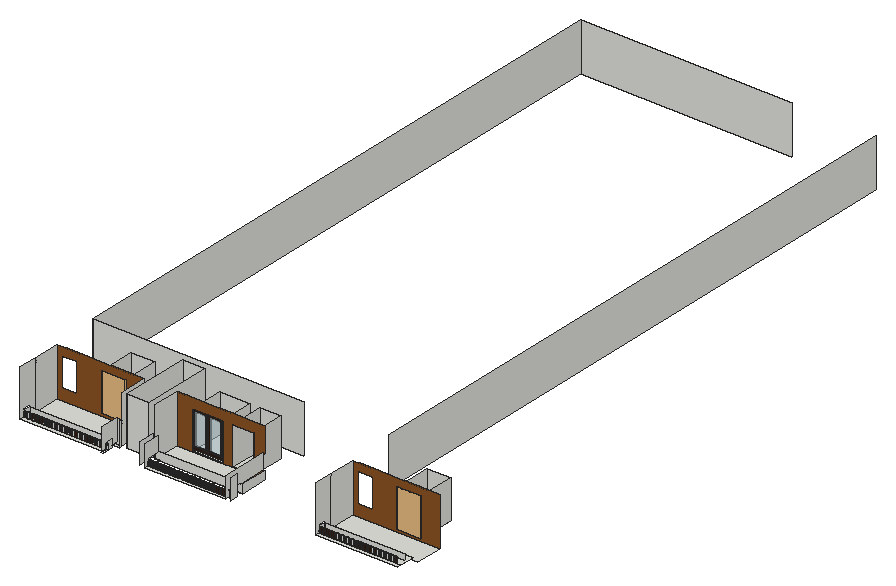
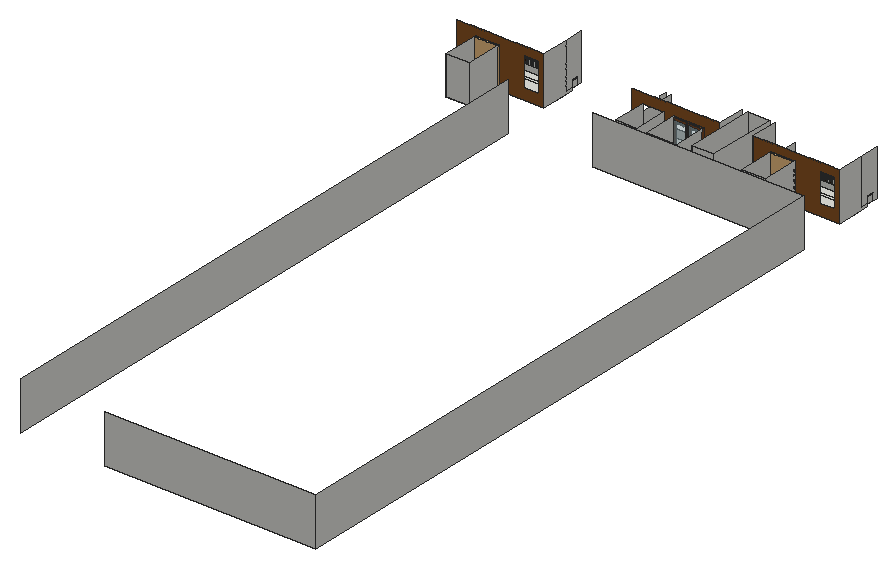
# SketchUp Ruby script. Lengths in inches.
U = 1.inch
M = Sketchup.active_model
def pt(a) = Geom::Point3d.new(a.map { |v| v * U })
def face(e, loops, mat)
  f = e.add_face(loops[0].map { |a| pt(a) })
  loops[1..].each { |l| e.add_face(l.map { |a| pt(a) }).erase! }
  f.material = f.back_material = mat if mat
  f
end
# faces: each face lists its corners as indices into pts; further lists are holes
def faces(e, pts, list, mat = nil) = list.each { |f| face(e, (f[0].is_a?(Array) ? f : [f]).map { |l| l.map { |i| pts[i] } }, mat) }
# xy, xz, yz: faces in a plane at the given z, y or x. An outline is a flat list of corners, or four numbers for a rectangle; further outlines are holes
def ring(l) = l.size == 4 ? [[l[0], l[1]], [l[2], l[1]], [l[2], l[3]], [l[0], l[3]]] : l.each_slice(2).to_a
def flat(e, list, mat, &to3) = list.each { |f| face(e, (f[0].is_a?(Array) ? f : [f]).map { |l| ring(l).map { |u, v| to3.(u, v) } }, mat) }
def xy(e, z, list, mat = nil) = flat(e, list, mat) { |x, y| [x, y, z] }
def xz(e, y, list, mat = nil) = flat(e, list, mat) { |x, z| [x, y, z] }
def yz(e, x, list, mat = nil) = flat(e, list, mat) { |y, z| [x, y, z] }
def lines(e, pts, list) = list.each { |a, b| e.add_line(pt(pts[a]), pt(pts[b])) }
# prism: a flat outline (further loops are holes) pulled along v
def prism(e, loops, v, mat = nil)
  f = face(e, loops, mat); d = Geom::Vector3d.new(v.map { |x| x * U })
  f.pushpull(f.normal.samedirection?(d) ? d.length : -d.length)
end
def box(e, o, s, mat = nil) = prism(e, [[o, [o[0] + s[0], o[1], o[2]], [o[0] + s[0], o[1] + s[1], o[2]], [o[0], o[1] + s[1], o[2]]]], [0, 0, s[2]], mat)
def at(x, y, z, deg = 0) = Geom::Transformation.translation(pt([x, y, z])) * Geom::Transformation.rotation(ORIGIN, Z_AXIS, deg.degrees)
def axes(o, x, y, z) = Geom::Transformation.new([*x, 0, *y, 0, *z, 0, *pt(o).to_a, 1])
def part(name) = M.definitions.add(name)
# library, detail: a bought-in or finely detailed component or shape, given as its bounding box
def library(name, o, s) = part(name).tap { |d| box(d.entities, o, s) }
def detail(e, o, s) = box(e.add_group.entities, o, s)
def put(e, d, t, mat = nil) = e.add_instance(d, t).tap { |i| i.material = mat if mat }
def group(e, t, mat = nil) = e.add_group.tap { |g| g.transformation = t; g.material = mat if mat }.entities
root = M.entities
M.materials.add("[Translucent Glass Safety]").color = [204, 235, 244]
M.materials["[Translucent Glass Safety]"].alpha = 0.5
M.materials.add("[Wood Floor Parquet]").color = [140, 85, 37]
M.materials.add("[Wood Veneer 01]").color = [51, 28, 15]
M.materials.add("[Wood Veneer 01]1").color = [120, 70, 37]
c1 = library("元件\#5",[-4.39,0,0],[5.37,35.83,90.55])
c2 = part("Component\#1")
xy(c2.entities,0,[[0,0,6,48]],"[Wood Veneer 01]1")
xy(c2.entities,4,[[0,4,1.8125,44],[1.8125,4,6,44]])
xy(c2.entities,80,[[0,4,1.8125,44],[1.8125,4,6,44]])
xy(c2.entities,84,[[0,0,6,48]],"[Wood Veneer 01]1")
xz(c2.entities,0,[[0,0,6,84]],"[Wood Veneer 01]1")
xz(c2.entities,4,[[0,4,1.8125,80],[1.8125,4,6,80]])
xz(c2.entities,44,[[0,4,1.8125,80],[1.8125,4,6,80]])
xz(c2.entities,48,[[0,0,6,84]],"[Wood Veneer 01]1")
yz(c2.entities,0,[[[0,0,48,84],[4,4,44,80]]],"[Wood Veneer 01]1")
yz(c2.entities,1.8125,[[4,4,44,80]],"[Translucent Glass Safety]")
yz(c2.entities,6,[[[0,0,48,84],[4,4,44,80]]],"[Wood Veneer 01]")
c3 = part("Group\#3")
put(c3.entities,c2,at(0,0,0),"[Wood Veneer 01]")
g1 = group(c3.entities,at(0,48,0),"[Wood Veneer 01]")
xy(g1,0,[[0,0,6,48]],"[Wood Veneer 01]1")
xy(g1,4,[[0,4,1.8125,44],[1.8125,4,6,44]])
xy(g1,80,[[0,4,1.8125,44],[1.8125,4,6,44]])
xy(g1,84,[[0,0,6,48]],"[Wood Veneer 01]1")
xz(g1,0,[[0,0,6,84]],"[Wood Veneer 01]1")
xz(g1,4,[[0,4,1.8125,80],[1.8125,4,6,80]])
xz(g1,44,[[0,4,1.8125,80],[1.8125,4,6,80]])
xz(g1,48,[[0,0,6,84]],"[Wood Veneer 01]1")
yz(g1,0,[[[0,0,48,84],[4,4,44,80]]],"[Wood Veneer 01]1")
yz(g1,1.8125,[[4,4,44,80]],"[Translucent Glass Safety]")
yz(g1,6,[[[0,0,48,84],[4,4,44,80]]],"[Wood Veneer 01]")
xy(root,134.6875,[[100.18,275.15,298.48,293.45],[833.74,275.15,1032.04,293.45],[298.48,286.21,315.43,293.45],[100.18,293.45,315.43,361.27],[328.03,293.45,382.74,465.02],
  [396.57,293.45,614.76,361.27],[833.74,293.45,1049,361.27]])
xy(root,135.5625,[[435.49,361.27,509.74,445.08],[534.92,361.27,587.67,445.08]])
xy(root,140.625,[[100.18,246.64,303.35,256.84],[409.32,246.64,609.07,246.64,609.07,256.84,412.47,256.84,412.47,255.72,409.32,255.72],[833.74,246.64,1036.91,256.84],[100.18,256.84,303.35,256.84,303.35,293.45,298.48,293.45,298.48,293.46,100.18,293.46],[833.74,256.84,1036.91,256.84,1036.91,293.45,1032.04,293.45,1032.04,293.46,833.74,293.46]])
xy(root,140.625,[[409.32,255.72,412.47,256.78]],"[Wood Veneer 01]")
xy(root,141,[[210.43,361.27,269.1,452.7],[943.99,361.27,1002.66,452.7]])
xz(root,255.72,[[409.32,140.625,412.47,154.75],[413.32,140.625,416.47,154.75],[417.32,140.625,420.47,154.75],[421.32,140.625,424.47,154.75],[425.32,140.625,428.47,154.75],
  [429.32,140.625,432.47,154.75],[433.32,140.625,436.47,154.75],[437.32,140.625,440.47,154.75],[441.32,140.625,444.47,154.75],[445.32,140.625,448.47,154.75],
  [449.32,140.625,452.47,154.75],[453.32,140.625,456.47,154.75],[457.32,140.625,460.47,154.75],[461.32,140.625,464.47,154.75],[465.32,140.625,468.47,154.75],
  [469.32,140.625,472.47,154.75],[473.32,140.625,476.47,154.75],[477.32,140.625,480.47,154.75],[481.32,140.625,484.47,154.75],[485.32,140.625,488.47,154.75],
  [489.32,140.625,492.47,154.75],[493.32,140.625,496.47,154.75],[497.32,140.625,500.47,154.75],[501.32,140.625,504.47,154.75],[505.32,140.625,508.47,154.75],
  [509.32,140.625,512.47,154.75],[513.32,140.625,516.47,154.75],[517.32,140.625,520.47,154.75],[521.32,140.625,524.47,154.75],[525.32,140.625,528.47,154.75],
  [529.32,140.625,532.47,154.75],[533.32,140.625,536.47,154.75],[537.32,140.625,540.47,154.75],[541.32,140.625,544.47,154.75],[545.32,140.625,548.47,154.75],
  [549.32,140.625,552.47,154.75],[553.32,140.625,556.47,154.75],[557.32,140.625,560.47,154.75],[561.32,140.625,564.47,154.75],[565.32,140.625,568.47,154.75],
  [569.32,140.625,572.47,154.75],[573.32,140.625,576.47,154.75],[577.32,140.625,580.47,154.75],[581.32,140.625,584.47,154.75],[585.32,140.625,588.47,154.75],
  [589.32,140.625,592.47,154.75],[593.32,140.625,596.47,154.75],[597.32,140.625,600.47,154.75],[601.32,140.625,604.47,154.75],[605.32,140.625,608.47,154.75],
  [609.32,140.625,612.47,154.75]],"[Wood Veneer 01]")
xz(root,256.78,[[409.32,140.625,412.47,154.75]],"[Wood Veneer 01]")
xz(root,256.84,[[103.45,140.625,104.3,154.75],[107.58,140.625,108.43,154.75],[111.7,140.625,112.55,154.75],[115.83,140.625,116.68,154.75],[119.95,140.625,120.8,154.75],
  [124.08,140.625,124.93,154.75],[128.2,140.625,129.05,154.75],[132.33,140.625,133.18,154.75],[136.45,140.625,137.3,154.75],[140.58,140.625,141.43,154.75],
  [144.7,140.625,145.55,154.75],[148.83,140.625,149.68,154.75],[152.95,140.625,153.8,154.75],[157.08,140.625,157.93,154.75],[161.2,140.625,162.05,154.75],
  [165.33,140.625,166.18,154.75],[169.45,140.625,170.3,154.75],[173.58,140.625,174.43,154.75],[177.7,140.625,178.55,154.75],[181.83,140.625,182.68,154.75],
  [185.95,140.625,186.8,154.75],[190.08,140.625,190.93,154.75],[194.2,140.625,195.05,154.75],[198.33,140.625,199.18,154.75],[202.45,140.625,203.3,154.75],
  [206.58,140.625,207.43,154.75],[210.7,140.625,211.55,154.75],[214.83,140.625,215.68,154.75],[218.95,140.625,219.8,154.75],[223.08,140.625,223.93,154.75],
  [227.2,140.625,228.05,154.75],[231.33,140.625,232.18,154.75],[235.45,140.625,236.3,154.75],[239.58,140.625,240.43,154.75],[243.7,140.625,244.55,154.75],
  [247.83,140.625,248.68,154.75],[251.95,140.625,252.8,154.75],[256.08,140.625,256.93,154.75],[260.2,140.625,261.05,154.75],[264.33,140.625,265.18,154.75],
  [268.45,140.625,269.3,154.75],[272.58,140.625,273.43,154.75],[276.7,140.625,277.55,154.75],[280.83,140.625,281.68,154.75],[284.95,140.625,285.8,154.75],
  [289.08,140.625,289.93,154.75],[293.2,140.625,294.05,154.75],[297.33,140.625,298.18,154.75],[301.45,140.625,302.3,154.75],[303.41,140.625,305.58,154.75],
  [306.43,140.625,309.7,154.75],[412.47,140.625,609.07,154.75],[609.07,140.625,614.76,154.75],[837.02,140.625,837.86,154.75],[841.14,140.625,841.99,154.75],
  [845.27,140.625,846.11,154.75],[849.39,140.625,850.24,154.75],[853.52,140.625,854.36,154.75],[857.64,140.625,858.49,154.75],[861.77,140.625,862.61,154.75],
  [865.89,140.625,866.74,154.75],[870.02,140.625,870.86,154.75],[874.14,140.625,874.99,154.75],[878.27,140.625,879.11,154.75],[882.39,140.625,883.24,154.75],
  [886.52,140.625,887.36,154.75],[890.64,140.625,891.49,154.75],[894.77,140.625,895.61,154.75],[898.89,140.625,899.74,154.75],[903.02,140.625,903.86,154.75],
  [907.14,140.625,907.99,154.75],[911.27,140.625,912.11,154.75],[915.39,140.625,916.24,154.75],[919.52,140.625,920.36,154.75],[923.64,140.625,924.49,154.75],
  [927.77,140.625,928.61,154.75],[931.89,140.625,932.74,154.75],[936.02,140.625,936.86,154.75],[940.14,140.625,940.99,154.75],[944.27,140.625,945.11,154.75],
  [948.39,140.625,949.24,154.75],[952.52,140.625,953.36,154.75],[956.64,140.625,957.49,154.75],[960.77,140.625,961.61,154.75],[964.89,140.625,965.74,154.75],
  [969.02,140.625,969.86,154.75],[973.14,140.625,973.99,154.75],[977.27,140.625,978.11,154.75],[981.39,140.625,982.24,154.75],[985.52,140.625,986.36,154.75],
  [989.64,140.625,990.49,154.75],[993.77,140.625,994.61,154.75],[997.89,140.625,998.74,154.75],[1002.02,140.625,1002.86,154.75],[1006.14,140.625,1006.99,154.75],
  [1010.27,140.625,1011.11,154.75],[1014.39,140.625,1015.24,154.75],[1018.52,140.625,1019.36,154.75],[1022.64,140.625,1023.49,154.75]])
xz(root,256.84,[[100.18,140.625,103.45,154.75],[104.3,140.625,107.58,154.75],[108.43,140.625,111.7,154.75],[112.55,140.625,115.83,154.75],[116.68,140.625,119.95,154.75],
  [120.8,140.625,124.08,154.75],[124.93,140.625,128.2,154.75],[129.05,140.625,132.33,154.75],[133.18,140.625,136.45,154.75],[137.3,140.625,140.58,154.75],
  [141.43,140.625,144.7,154.75],[145.55,140.625,148.83,154.75],[149.68,140.625,152.95,154.75],[153.8,140.625,157.08,154.75],[157.93,140.625,161.2,154.75],
  [162.05,140.625,165.33,154.75],[166.18,140.625,169.45,154.75],[170.3,140.625,173.58,154.75],[174.43,140.625,177.7,154.75],[178.55,140.625,181.83,154.75],
  [182.68,140.625,185.95,154.75],[186.8,140.625,190.08,154.75],[190.93,140.625,194.2,154.75],[195.05,140.625,198.33,154.75],[199.18,140.625,202.45,154.75],
  [203.3,140.625,206.58,154.75],[207.43,140.625,210.7,154.75],[211.55,140.625,214.83,154.75],[215.68,140.625,218.95,154.75],[219.8,140.625,223.08,154.75],
  [223.93,140.625,227.2,154.75],[228.05,140.625,231.33,154.75],[232.18,140.625,235.45,154.75],[236.3,140.625,239.58,154.75],[240.43,140.625,243.7,154.75],
  [244.55,140.625,247.83,154.75],[248.68,140.625,251.95,154.75],[252.8,140.625,256.08,154.75],[256.93,140.625,260.2,154.75],[261.05,140.625,264.33,154.75],
  [265.18,140.625,268.45,154.75],[269.3,140.625,272.58,154.75],[273.43,140.625,276.7,154.75],[277.55,140.625,280.83,154.75],[281.68,140.625,284.95,154.75],
  [285.8,140.625,289.08,154.75],[289.93,140.625,293.2,154.75],[294.05,140.625,297.33,154.75],[298.18,140.625,301.45,154.75],[302.3,140.625,303.41,154.75],
  [833.74,140.625,837.02,154.75],[837.86,140.625,841.14,154.75],[841.99,140.625,845.27,154.75],[846.11,140.625,849.39,154.75],[850.24,140.625,853.52,154.75],
  [854.36,140.625,857.64,154.75],[858.49,140.625,861.77,154.75],[862.61,140.625,865.89,154.75],[866.74,140.625,870.02,154.75],[870.86,140.625,874.14,154.75],
  [874.99,140.625,878.27,154.75],[879.11,140.625,882.39,154.75],[883.24,140.625,886.52,154.75],[887.36,140.625,890.64,154.75],[891.49,140.625,894.77,154.75],
  [895.61,140.625,898.89,154.75],[899.74,140.625,903.02,154.75],[903.86,140.625,907.14,154.75],[907.99,140.625,911.27,154.75],[912.11,140.625,915.39,154.75],
  [916.24,140.625,919.52,154.75],[920.36,140.625,923.64,154.75],[924.49,140.625,927.77,154.75],[928.61,140.625,931.89,154.75],[932.74,140.625,936.02,154.75],
  [936.86,140.625,940.14,154.75],[940.99,140.625,944.27,154.75],[945.11,140.625,948.39,154.75],[949.24,140.625,952.52,154.75],[953.36,140.625,956.64,154.75],
  [957.49,140.625,960.77,154.75],[961.61,140.625,964.89,154.75],[965.74,140.625,969.02,154.75],[969.86,140.625,973.14,154.75],[973.99,140.625,977.27,154.75],
  [978.11,140.625,981.39,154.75],[982.24,140.625,985.52,154.75],[986.36,140.625,989.64,154.75],[990.49,140.625,993.77,154.75],[994.61,140.625,997.89,154.75],
  [998.74,140.625,1002.02,154.75],[1002.86,140.625,1006.14,154.75],[1006.99,140.625,1010.27,154.75],[1011.11,140.625,1014.39,154.75],[1015.24,140.625,1018.52,154.75],
  [1019.36,140.625,1022.64,154.75],[1023.49,140.625,1026.77,154.75]],"[Wood Veneer 01]")
xz(root,266.43,[[614.76,140.625,622,154.75]])
xz(root,275.15,[[100.18,134.6875,298.48,154.75],[298.48,134.6875,303.41,154.75],[833.74,134.6875,1032.04,154.75]])
xz(root,293.45,[[298.48,134.6875,298.48,140.625,303.35,140.625,303.35,193,315.43,193,315.43,134.6875],[328.03,134.6875,382.74,254.6875],[396.57,134.6875,614.76,154.75]])
xz(root,361.27,[[435.49,134.6875,509.74,135.5625],[534.92,134.6875,587.67,135.5625]])
xz(root,361.27,[[[100.18,134.6875,315.43,134.6875,315.43,253.5625,310.68,253.5625,310.68,254.6875,309.43,254.6875,309.43,253.5625,304.68,253.5625,304.68,254.6875,303.43,254.6875,303.43,253.5625,298.68,253.5625,298.68,254.6875,297.43,254.6875,297.43,253.5625,292.68,253.5625,292.68,254.6875,291.43,254.6875,291.43,253.5625,286.68,253.5625,286.68,254.6875,285.43,254.6875,285.43,253.5625,280.68,253.5625,280.68,254.6875,279.43,254.6875,279.43,253.5625,274.68,253.5625,274.68,254.6875,273.43,254.6875,273.43,253.5625,268.68,253.5625,268.68,254.6875,267.43,254.6875,267.43,253.5625,262.68,253.5625,262.68,254.6875,261.43,254.6875,261.43,253.5625,256.68,253.5625,256.68,254.6875,255.43,254.6875,255.43,253.875,250.68,253.875,250.68,254.6875,249.43,254.6875,249.43,253.875,244.68,253.875,244.68,254.6875,243.43,254.6875,243.43,253.9375,238.68,253.9375,238.68,254.6875,237.43,254.6875,237.43,253.9375,232.68,253.9375,232.68,254.6875,231.43,254.6875,231.43,253.9375,226.68,253.9375,226.68,254.6875,225.43,254.6875,225.43,253.9375,220.68,253.9375,220.68,254.6875,219.43,254.6875,219.43,253.9375,214.68,253.9375,214.68,254.6875,213.43,254.6875,213.43,253.9375,208.68,253.9375,208.68,254.6875,207.43,254.6875,207.43,253.9375,202.68,253.9375,202.68,254.6875,201.43,254.6875,201.43,253.9375,196.68,253.9375,196.68,254.6875,195.43,254.6875,195.43,253.9375,190.68,253.9375,190.68,254.6875,189.43,254.6875,189.43,253.9375,184.68,253.9375,184.68,254.6875,183.43,254.6875,183.43,253.9375,178.68,253.9375,178.68,254.6875,177.43,254.6875,177.43,253.9375,172.68,253.9375,172.68,254.6875,171.43,254.6875,171.43,253.9375,166.68,253.9375,166.68,254.6875,165.43,254.6875,165.43,253.9375,160.68,253.9375,160.68,254.6875,159.43,254.6875,159.43,253.9375,154.68,253.9375,154.68,254.6875,153.43,254.6875,153.43,253.9375,148.68,253.9375,148.68,254.6875,147.43,254.6875,147.43,253.9375,142.68,253.9375,142.68,254.6875,141.43,254.6875,141.43,253.9375,136.68,253.9375,136.68,254.6875,135.43,254.6875,135.43,253.9375,130.68,253.9375,130.68,254.6875,129.43,254.6875,129.43,253.9375,124.68,253.9375,124.68,254.6875,123.43,254.6875,123.43,253.9375,118.68,253.9375,118.68,254.6875,117.43,254.6875,117.43,253.9375,112.68,253.9375,112.68,254.6875,100.18,254.6875],[210.43,141,269.1,235.92],[111.92,162.74,149.24,234.87]],[396.57,134.6875,435.49,134.6875,435.49,230.0625,509.74,230.0625,509.74,134.6875,534.92,134.6875,534.92,230.125,587.67,230.125,587.67,134.6875,614.76,134.6875,614.76,154.75,609.07,154.75,609.07,193,614.76,193,614.76,253.9375,612.57,253.9375,612.57,254.6875,610.96,254.6875,610.96,253.9375,606.57,253.9375,606.57,254.6875,604.96,254.6875,604.96,253.9375,600.57,253.9375,600.57,254.6875,598.96,254.6875,598.96,253.9375,594.57,253.9375,594.57,254.6875,592.96,254.6875,592.96,253.9375,588.57,253.9375,588.57,254.6875,586.96,254.6875,586.96,253.9375,582.57,253.9375,582.57,254.6875,580.96,254.6875,580.96,253.9375,576.57,253.9375,576.57,254.6875,574.96,254.6875,574.96,253.9375,570.57,253.9375,570.57,254.6875,568.96,254.6875,568.96,253.9375,564.57,253.9375,564.57,254.6875,562.96,254.6875,562.96,253.9375,558.57,253.9375,558.57,254.6875,556.96,254.6875,556.96,253.9375,552.57,253.9375,552.57,254.6875,550.96,254.6875,550.96,253.9375,546.57,253.9375,546.57,254.6875,544.96,254.6875,544.96,253.9375,540.57,253.9375,540.57,254.6875,538.96,254.6875,538.96,253.9375,534.57,253.9375,534.57,254.6875,532.96,254.6875,532.96,253.9375,528.57,253.9375,528.57,254.6875,526.96,254.6875,526.96,253.9375,522.57,253.9375,522.57,254.6875,520.96,254.6875,520.96,253.9375,516.57,253.9375,516.57,254.6875,514.96,254.6875,514.96,253.9375,510.57,253.9375,510.57,254.6875,508.96,254.6875,508.96,253.9375,504.57,253.9375,504.57,254.6875,502.96,254.6875,502.96,253.9375,498.57,253.9375,498.57,254.6875,496.96,254.6875,496.96,253.9375,492.57,253.9375,492.57,254.6875,490.96,254.6875,490.96,253.9375,486.57,253.9375,486.57,254.6875,484.96,254.6875,484.96,253.9375,480.57,253.9375,480.57,254.6875,478.96,254.6875,478.96,253.9375,474.57,253.9375,474.57,254.6875,472.96,254.6875,472.96,253.9375,468.57,253.9375,468.57,254.6875,466.96,254.6875,466.96,253.9375,462.57,253.9375,462.57,254.6875,460.96,254.6875,460.96,253.9375,456.57,253.9375,456.57,254.6875,454.96,254.6875,454.96,253.9375,450.57,253.9375,450.57,254.6875,448.96,254.6875,448.96,253.9375,444.57,253.9375,444.57,254.6875,442.96,254.6875,442.96,253.9375,438.57,253.9375,438.57,254.6875,436.96,254.6875,436.96,253.9375,432.57,253.9375,432.57,254.6875,430.96,254.6875,430.96,253.9375,426.57,253.9375,426.57,254.6875,424.96,254.6875,424.96,253.9375,420.57,253.9375,420.57,254.6875,418.96,254.6875,418.96,253.9375,414.57,253.9375,414.57,254.6875,412.96,254.6875,412.96,253.9375,408.57,253.9375,408.57,254.6875,406.96,254.6875,406.96,253.9375,402.57,253.9375,402.57,254.6875,400.96,254.6875,400.96,253.9375,396.57,253.9375],[[833.74,134.6875,1049,134.6875,1049,253.5625,1044.25,253.5625,1044.25,254.6875,1043,254.6875,1043,253.5625,1038.25,253.5625,1038.25,254.6875,1037,254.6875,1037,253.5625,1032.25,253.5625,1032.25,254.6875,1031,254.6875,1031,253.5625,1026.25,253.5625,1026.25,254.6875,1025,254.6875,1025,253.5625,1020.25,253.5625,1020.25,254.6875,1019,254.6875,1019,253.5625,1014.25,253.5625,1014.25,254.6875,1013,254.6875,1013,253.5625,1008.25,253.5625,1008.25,254.6875,1007,254.6875,1007,253.5625,1002.25,253.5625,1002.25,254.6875,1001,254.6875,1001,253.5625,996.25,253.5625,996.25,254.6875,995,254.6875,995,253.5625,990.25,253.5625,990.25,254.6875,989,254.6875,989,253.875,984.25,253.875,984.25,254.6875,983,254.6875,983,253.875,978.25,253.875,978.25,254.6875,977,254.6875,977,253.9375,972.25,253.9375,972.25,254.6875,971,254.6875,971,253.9375,966.25,253.9375,966.25,254.6875,965,254.6875,965,253.9375,960.25,253.9375,960.25,254.6875,959,254.6875,959,253.9375,954.25,253.9375,954.25,254.6875,953,254.6875,953,253.9375,948.25,253.9375,948.25,254.6875,947,254.6875,947,253.9375,942.25,253.9375,942.25,254.6875,941,254.6875,941,253.9375,936.25,253.9375,936.25,254.6875,935,254.6875,935,253.9375,930.25,253.9375,930.25,254.6875,929,254.6875,929,253.9375,924.25,253.9375,924.25,254.6875,923,254.6875,923,253.9375,918.25,253.9375,918.25,254.6875,917,254.6875,917,253.9375,912.25,253.9375,912.25,254.6875,911,254.6875,911,253.9375,906.25,253.9375,906.25,254.6875,905,254.6875,905,253.9375,900.25,253.9375,900.25,254.6875,899,254.6875,899,253.9375,894.25,253.9375,894.25,254.6875,893,254.6875,893,253.9375,888.25,253.9375,888.25,254.6875,887,254.6875,887,253.9375,882.25,253.9375,882.25,254.6875,881,254.6875,881,253.9375,876.25,253.9375,876.25,254.6875,875,254.6875,875,253.9375,870.25,253.9375,870.25,254.6875,869,254.6875,869,253.9375,864.25,253.9375,864.25,254.6875,863,254.6875,863,253.9375,858.25,253.9375,858.25,254.6875,857,254.6875,857,253.9375,852.25,253.9375,852.25,254.6875,851,254.6875,851,253.9375,846.25,253.9375,846.25,254.6875,833.74,254.6875],[943.99,141,1002.66,235.92],[845.49,162.74,882.8,234.87]]],"[Wood Floor Parquet]")
xz(root,445.08,[[435.49,135.5625,509.74,230.0625],[534.92,135.5625,587.67,230.125]])
xz(root,452.7,[[210.43,141,269.1,235.92],[943.99,141,1002.66,235.92]])
xz(root,465.02,[[328.03,134.6875,382.74,254.6875]])
xz(root,483.79,[[90.36,134.6875,614.76,254.6875]])
xz(root,1996.66,[[90.36,134.6875,614.76,254.6875]])
yz(root,90.36,[[483.79,134.6875,1996.66,254.6875]])
yz(root,100.18,[[275.15,134.6875,361.27,134.6875,361.27,254.6875,293.46,254.6875,293.46,140.625,275.15,140.625],[246.64,140.625,256.84,140.625,256.84,154.75,254.22,154.75,254.22,158.1875,275.15,158.1875,275.15,140.625,293.46,140.625,293.46,254.6875,246.64,254.6875],[256.84,140.625,275.15,154.75]])
yz(root,210.43,[[361.27,141,452.7,235.92]])
yz(root,269.1,[[361.27,141,452.7,235.92]])
yz(root,303.35,[[246.64,140.625,293.45,193]])
yz(root,303.41,[[256.84,134.6875,275.15,154.75]])
yz(root,315.43,[[286.21,134.6875,293.45,193],[293.45,134.6875,293.46,193],[293.46,134.6875,293.46,193,293.45,193,293.45,253.5625,361.27,253.5625,361.27,134.6875]])
yz(root,328.03,[[293.45,134.6875,465.02,254.6875]])
yz(root,382.74,[[293.45,134.6875,465.02,254.6875]])
yz(root,396.57,[[293.45,134.6875,361.27,253.9375],[246.64,141.6875,286.21,193]])
yz(root,409.32,[[246.64,140.625,255.72,140.625,255.72,154.75,254.22,154.75,254.22,156.9375,286.21,156.9375,286.21,193,246.64,193]])
yz(root,409.32,[[255.72,140.625,256.78,154.75]],"[Wood Veneer 01]")
yz(root,412.47,[[255.72,140.625,256.78,154.75],[256.78,140.625,256.84,154.75]],"[Wood Veneer 01]")
yz(root,416.47,[[255.72,140.625,256.78,154.75]],"[Wood Veneer 01]")
yz(root,420.47,[[255.72,140.625,256.78,154.75]],"[Wood Veneer 01]")
yz(root,424.47,[[255.72,140.625,256.78,154.75]],"[Wood Veneer 01]")
yz(root,428.47,[[255.72,140.625,256.78,154.75]],"[Wood Veneer 01]")
yz(root,432.47,[[255.72,140.625,256.78,154.75]],"[Wood Veneer 01]")
yz(root,435.49,[[361.27,135.5625,445.08,230.0625]])
yz(root,436.47,[[255.72,140.625,256.78,154.75]],"[Wood Veneer 01]")
yz(root,440.47,[[255.72,140.625,256.78,154.75]],"[Wood Veneer 01]")
yz(root,444.47,[[255.72,140.625,256.78,154.75]],"[Wood Veneer 01]")
yz(root,448.47,[[255.72,140.625,256.78,154.75]],"[Wood Veneer 01]")
yz(root,452.47,[[255.72,140.625,256.78,154.75]],"[Wood Veneer 01]")
yz(root,456.47,[[255.72,140.625,256.78,154.75]],"[Wood Veneer 01]")
yz(root,460.47,[[255.72,140.625,256.78,154.75]],"[Wood Veneer 01]")
yz(root,464.47,[[255.72,140.625,256.78,154.75]],"[Wood Veneer 01]")
yz(root,468.47,[[255.72,140.625,256.78,154.75]],"[Wood Veneer 01]")
yz(root,472.47,[[255.72,140.625,256.78,154.75]],"[Wood Veneer 01]")
yz(root,476.47,[[255.72,140.625,256.78,154.75]],"[Wood Veneer 01]")
yz(root,480.47,[[255.72,140.625,256.78,154.75]],"[Wood Veneer 01]")
yz(root,484.47,[[255.72,140.625,256.78,154.75]],"[Wood Veneer 01]")
yz(root,488.47,[[255.72,140.625,256.78,154.75]],"[Wood Veneer 01]")
yz(root,492.47,[[255.72,140.625,256.78,154.75]],"[Wood Veneer 01]")
yz(root,496.47,[[255.72,140.625,256.78,154.75]],"[Wood Veneer 01]")
yz(root,500.47,[[255.72,140.625,256.78,154.75]],"[Wood Veneer 01]")
yz(root,504.47,[[255.72,140.625,256.78,154.75]],"[Wood Veneer 01]")
yz(root,508.47,[[255.72,140.625,256.78,154.75]],"[Wood Veneer 01]")
yz(root,509.74,[[361.27,135.5625,445.08,230.0625]])
yz(root,512.47,[[255.72,140.625,256.78,154.75]],"[Wood Veneer 01]")
yz(root,516.47,[[255.72,140.625,256.78,154.75]],"[Wood Veneer 01]")
yz(root,520.47,[[255.72,140.625,256.78,154.75]],"[Wood Veneer 01]")
yz(root,524.47,[[255.72,140.625,256.78,154.75]],"[Wood Veneer 01]")
yz(root,528.47,[[255.72,140.625,256.78,154.75]],"[Wood Veneer 01]")
yz(root,532.47,[[255.72,140.625,256.78,154.75]],"[Wood Veneer 01]")
yz(root,534.92,[[361.27,135.5625,445.08,230.125]])
yz(root,536.47,[[255.72,140.625,256.78,154.75]],"[Wood Veneer 01]")
yz(root,540.47,[[255.72,140.625,256.78,154.75]],"[Wood Veneer 01]")
yz(root,544.47,[[255.72,140.625,256.78,154.75]],"[Wood Veneer 01]")
yz(root,548.47,[[255.72,140.625,256.78,154.75]],"[Wood Veneer 01]")
yz(root,552.47,[[255.72,140.625,256.78,154.75]],"[Wood Veneer 01]")
yz(root,556.47,[[255.72,140.625,256.78,154.75]],"[Wood Veneer 01]")
yz(root,560.47,[[255.72,140.625,256.78,154.75]],"[Wood Veneer 01]")
yz(root,564.47,[[255.72,140.625,256.78,154.75]],"[Wood Veneer 01]")
yz(root,568.47,[[255.72,140.625,256.78,154.75]],"[Wood Veneer 01]")
yz(root,572.47,[[255.72,140.625,256.78,154.75]],"[Wood Veneer 01]")
yz(root,587.67,[[361.27,135.5625,445.08,230.125]])
yz(root,609.07,[[246.64,140.625,246.64,193,361.27,193,361.27,154.75,293.45,154.75,293.45,156.9375,254.22,156.9375,254.22,154.75,256.84,154.75,256.84,140.625]])
yz(root,614.76,[[293.45,134.6875,361.27,154.75],[256.84,140.625,266.43,154.75]])
yz(root,622,[[246.64,140.625,266.43,193]])
yz(root,823.93,[[483.79,134.6875,1996.66,254.6875]])
yz(root,833.74,[[275.15,134.6875,361.27,134.6875,361.27,254.6875,293.46,254.6875,293.46,140.625,275.15,140.625],[246.64,140.625,256.84,140.625,256.84,154.75,254.22,154.75,254.22,158.1875,275.15,158.1875,275.15,140.625,293.46,140.625,293.46,254.6875,246.64,254.6875],[256.84,140.625,275.15,154.75]])
yz(root,943.99,[[361.27,141,452.7,235.92]])
yz(root,1002.66,[[361.27,141,452.7,235.92]])
p = [[298.48,275.15,140.625],[303.35,275.15,140.625],[298.48,275.15,134.6875],[298.48,246.64,134.6875],[303.41,256.84,134.6875],[303.41,246.64,134.6875],
  [415.64,266.43,141.6875],[415.64,286.21,141.6875],[396.57,286.21,141.6875],[588.47,256.78,140.625],[588.47,255.72,140.625],[592.47,256.78,140.625],
  [592.47,256.78,154.75],[576.47,256.78,140.625],[576.47,255.72,140.625],[584.47,256.78,140.625],[584.47,255.72,140.625],[580.47,256.78,140.625],
  [580.47,256.78,154.75],[588.47,256.78,154.75],[576.47,256.78,154.75],[580.47,255.72,140.625],[584.47,256.78,154.75],[596.47,256.78,140.625],
  [596.47,255.72,140.625],[596.47,256.78,154.75],[592.47,255.72,140.625],[604.47,256.78,140.625],[604.47,256.78,154.75],[600.47,256.78,140.625],
  [600.47,255.72,140.625],[600.47,256.78,154.75],[612.47,256.78,140.625],[612.47,256.78,154.75],[608.47,256.78,140.625],[608.47,255.72,140.625],
  [604.47,255.72,140.625],[608.47,256.78,154.75],[612.47,255.72,140.625]]
lines(root,p,[[0,1],[2,3],[4,5],[6,7],[8,7],[9,10],[11,12],[13,14],[15,16],[17,18],[9,19],[13,20],
  [17,21],[15,22],[23,24],[23,25],[11,26],[27,28],[29,30],[29,31],[32,33],[34,35],[27,36],[34,37],
  [32,38]])
put(root,c1,axes([210.43,361.64,141],[0,-1,0],[1.63746,0,0],[0,0,1.04827]))
put(root,c3,axes([435.49,367.27,141.22],[0,-1,0],[0.77344,0,0],[0,0,1.0577]))
put(root,c1,axes([943.99,361.64,141],[0,-1,0],[1.63746,0,0],[0,0,1.04827]))
